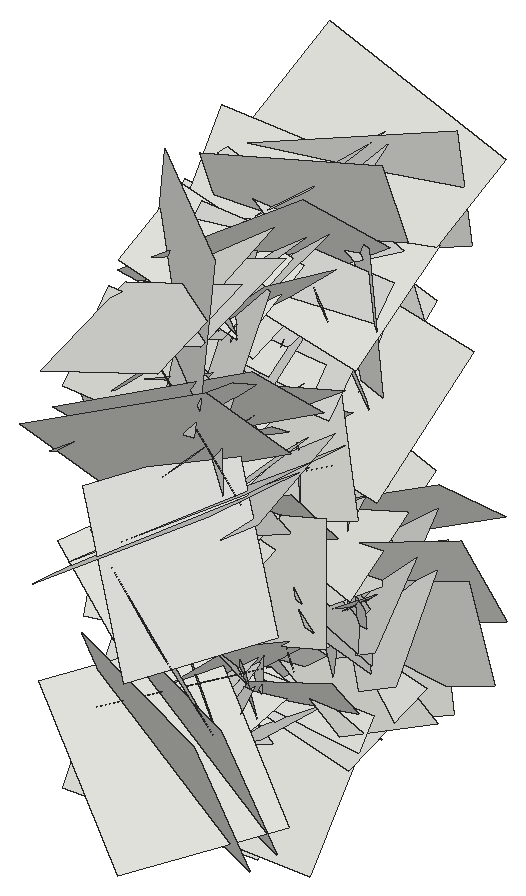
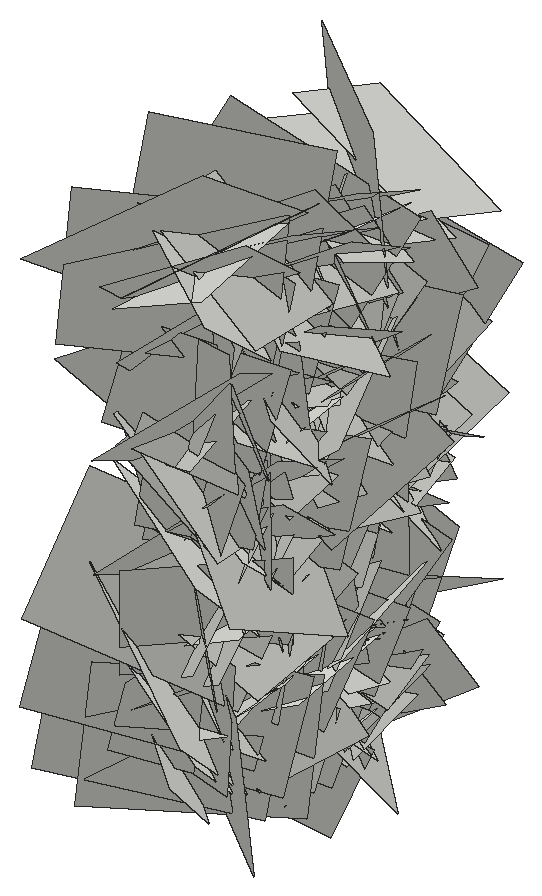
# SketchUp Ruby script. Lengths in inches.
U = 1.inch
M = Sketchup.active_model
def pt(a) = Geom::Point3d.new(a.map { |v| v * U })
def face(e, loops, mat)
  f = e.add_face(loops[0].map { |a| pt(a) })
  loops[1..].each { |l| e.add_face(l.map { |a| pt(a) }).erase! }
  f.material = f.back_material = mat if mat
  f
end
# faces: each face lists its corners as indices into pts; further lists are holes
def faces(e, pts, list, mat = nil) = list.each { |f| face(e, (f[0].is_a?(Array) ? f : [f]).map { |l| l.map { |i| pts[i] } }, mat) }
# xy, xz, yz: faces in a plane at the given z, y or x. An outline is a flat list of corners, or four numbers for a rectangle; further outlines are holes
def ring(l) = l.size == 4 ? [[l[0], l[1]], [l[2], l[1]], [l[2], l[3]], [l[0], l[3]]] : l.each_slice(2).to_a
def flat(e, list, mat, &to3) = list.each { |f| face(e, (f[0].is_a?(Array) ? f : [f]).map { |l| ring(l).map { |u, v| to3.(u, v) } }, mat) }
def xy(e, z, list, mat = nil) = flat(e, list, mat) { |x, y| [x, y, z] }
def xz(e, y, list, mat = nil) = flat(e, list, mat) { |x, z| [x, y, z] }
def yz(e, x, list, mat = nil) = flat(e, list, mat) { |y, z| [x, y, z] }
def lines(e, pts, list) = list.each { |a, b| e.add_line(pt(pts[a]), pt(pts[b])) }
# prism: a flat outline (further loops are holes) pulled along v
def prism(e, loops, v, mat = nil)
  f = face(e, loops, mat); d = Geom::Vector3d.new(v.map { |x| x * U })
  f.pushpull(f.normal.samedirection?(d) ? d.length : -d.length)
end
def box(e, o, s, mat = nil) = prism(e, [[o, [o[0] + s[0], o[1], o[2]], [o[0] + s[0], o[1] + s[1], o[2]], [o[0], o[1] + s[1], o[2]]]], [0, 0, s[2]], mat)
def at(x, y, z, deg = 0) = Geom::Transformation.translation(pt([x, y, z])) * Geom::Transformation.rotation(ORIGIN, Z_AXIS, deg.degrees)
def axes(o, x, y, z) = Geom::Transformation.new([*x, 0, *y, 0, *z, 0, *pt(o).to_a, 1])
def part(name) = M.definitions.add(name)
# library, detail: a bought-in or finely detailed component or shape, given as its bounding box
def library(name, o, s) = part(name).tap { |d| box(d.entities, o, s) }
def detail(e, o, s) = box(e.add_group.entities, o, s)
def put(e, d, t, mat = nil) = e.add_instance(d, t).tap { |i| i.material = mat if mat }
def group(e, t, mat = nil) = e.add_group.tap { |g| g.transformation = t; g.material = mat if mat }.entities
root = M.entities
c1 = part("Component\#6")
p = [[0.01,0,0],[0,3.24,4.54],[4.32,3.24,4.54],[4.33,0,0]]
faces(c1.entities,p,[[0,1,2,3]])
put(root,c1,axes([38.11,133.2,0.29],[0.16868,0.00753,1.30134],[0.16064,1.302,-0.02607],[-1.37005,0.15359,0.15716]))
put(root,c1,axes([34.14,134.57,7.51],[-0.06425,-0.0713,-0.65597],[0.02618,-0.65852,0.06929],[0.69893,0.01811,-0.0629]))
put(root,c1,axes([38.11,128.52,17.74],[-0.08604,0.43028,-0.81229],[-0.04293,-0.81633,-0.42838],[-0.97342,-0.00203,0.0907]))
put(root,c1,axes([34.14,132.11,13.83],[-0.12823,-0.67114,-0.46171],[-0.10246,-0.45164,0.68184],[0.85739,-0.15435,0.01243]))
put(root,c1,axes([38.11,133.79,15.82],[-0.11741,-0.82822,-0.37202],[-0.00882,-0.37384,0.83474],[-0.96237,0.10447,0.03774]))
put(root,c1,axes([34.14,131.53,3.64],[-0.03356,0.34972,-0.55611],[0.01458,-0.55628,-0.35061],[0.69619,0.02851,-0.01946]))
put(root,c1,axes([34.14,130.57,14.69],[-0.08088,0.56373,-0.36339],[0.06437,-0.35843,-0.56878],[0.70803,0.09698,0.0102]))
put(root,c1,axes([38.11,130.125,12.36],[0.14413,1.23778,0.56401],[0.30073,0.52855,-1.22835],[-1.41013,0.23923,-0.20431]))
put(root,c1,axes([38.11,129.28,18.375],[-0.15104,-0.37703,-0.77667],[0.00911,-0.78776,0.38083],[-0.9151,0.05438,0.13199]))
put(root,c1,axes([38.11,132.6,22.9],[-0.05818,0.99288,0.05669],[0.07779,0.06066,-0.99145],[-1.05129,-0.05046,-0.07649]))
put(root,c1,axes([34.14,133.3125,17.59],[0.01529,0.27468,0.5349],[0.08187,0.52978,-0.27413],[0.6321,-0.07526,0.02257]))
put(root,c1,axes([34.14,129.84,16.13],[0.05288,0.68465,0.04631],[-0.09068,0.05228,-0.68068],[0.72171,-0.04359,-0.08892]))
put(root,c1,axes([38.11,129.45,15.69],[0.00555,0.72683,0.86308],[0.19522,0.85097,-0.71774],[-1.18002,0.1442,-0.11468]))
put(root,c1,axes([34.14,129.41,10.95],[-0.18775,-0.48629,-0.69123],[0.00245,-0.70652,0.49646],[0.89586,-0.09998,-0.14623]))
put(root,c1,axes([34.14,132.63,6.14],[-0.10731,0.87556,-0.00554],[-0.12201,-0.01884,-0.87366],[0.92006,0.09962,-0.1165]))
put(root,c1,axes([38.11,133.96,12.5],[-0.03937,0.24323,0.81298],[-0.12274,0.80469,-0.24604],[-0.89109,-0.12158,-0.00203]))
put(root,c1,axes([38.11,127.6,6.32],[-0.09105,0.77875,-0.27248],[-0.08108,-0.28029,-0.77696],[-0.87078,-0.05533,0.10084]))
put(root,c1,axes([38.11,133.1,9.3125],[0.02086,0.87239,-0.16813],[-0.14049,-0.16341,-0.8634],[-0.93122,0.04419,0.12649]))
put(root,c1,axes([38.11,131.05,1.96],[0.03915,-1.05631,0.36623],[0.17317,0.36759,1.04378],[-1.17236,0.01903,0.16641]))
put(root,c1,axes([34.14,133.88,6.93],[-0.12434,-0.60409,0.41763],[0.12699,0.40152,0.61444],[0.76804,-0.16419,-0.03398]))
put(root,c1,axes([38.11,136.93,7.59],[0.11136,0.24127,-0.97313],[-0.07388,-0.97433,-0.24909],[-1.06018,0.09324,-0.08486]))
put(root,c1,axes([34.14,130.03,2.94],[-0.11679,-0.3481,0.76621],[-0.04914,0.77408,0.34502],[0.89071,-0.00294,0.1195]))
put(root,c1,axes([34.14,129.23,5.41],[-0.17398,-0.60139,0.60701],[0.02487,0.6147,0.61536],[0.9054,-0.13245,0.09973]))
put(root,c1,axes([38.11,132.5,3.06],[0.12033,-0.77552,-0.96336],[0.26418,-0.93322,0.78062],[-1.28404,-0.26468,0.07033]))
put(root,c1,axes([34.14,129.18,10.77],[0.08644,0.04023,-0.60323],[0.06997,-0.60565,-0.03147],[0.63702,0.06107,0.08531]))
put(root,c1,axes([38.11,132.55,10.48],[0.11298,-1.07137,-0.22101],[0.09706,-0.21254,1.07447],[-1.1555,-0.12261,0.06864]))
put(root,c1,axes([34.14,128.34,18.92],[0.04874,0.38349,0.62334],[-0.06251,0.62448,-0.37984],[0.77325,0.02631,-0.07]))
put(root,c1,axes([34.14,129.8,15.91],[0.05085,-0.71724,0.33006],[-0.13843,0.31891,0.71198],[0.82538,0.09767,0.09907]))
put(root,c1,axes([38.11,127.86,19.19],[0.25173,1.01088,0.57921],[0.04385,0.58343,-1.03521],[-1.23418,0.22691,0.08136]))
put(root,c1,axes([38.11,127.34,21.1],[0.03089,0.79811,0.32897],[-0.11706,0.3299,-0.79059],[-0.90753,-0.01539,0.11317]))
put(root,c1,axes([34.14,133.42,16.97],[-0.14677,0.94615,0.46149],[-0.22557,0.4307,-0.94687],[1.09283,0.21597,-0.13346]))
put(root,c1,axes([34.14,133.96,6.46],[-0.0893,0.11056,0.97068],[-0.19494,0.95507,-0.12474],[1.01706,0.19277,0.06132]))
put(root,c1,axes([38.11,136.53,11.26],[0.01536,-0.64622,-0.54667],[-0.11065,-0.54394,0.64022],[-0.89037,0.05645,-0.089]))
put(root,c1,axes([34.14,131.99,-0.9375],[0.0225,-0.54484,0.50649],[-0.02225,0.50605,0.54525],[0.78821,0.02984,0.00093]))
put(root,c1,axes([38.11,127.95,5.4],[-0.05879,0.74539,0.22064],[-0.10629,0.21249,-0.74307],[-0.81711,-0.08127,0.08079]))
put(root,c1,axes([34.14,125.86,8.82],[0.02658,0.53015,0.39509],[0.11889,0.38623,-0.52538],[0.69069,-0.08688,0.07523]))
put(root,c1,axes([34.14,131.86,3.01],[0.01467,-0.55248,-0.51034],[-0.00827,-0.51051,0.55244],[0.7972,0.00487,0.01512]))
put(root,c1,axes([34.14,136.82,15.87],[-0.16772,-0.74319,-0.48228],[0.03783,-0.49486,0.75087],[0.93836,-0.11289,-0.11647]))
put(root,c1,axes([38.11,125.93,11.7],[-0.16945,0.67455,-0.05214],[-0.09647,-0.07453,-0.68517],[-0.71064,-0.15073,0.10544]))
put(root,c1,axes([38.11,127.92,4.7],[-0.092,0.70183,0.2556],[-0.07294,0.24871,-0.70628],[-0.78837,-0.10491,0.03552]))
put(root,c1,axes([38.11,128.53,16.93],[0.30517,1.08519,-0.55956],[0.1011,-0.59314,-1.10124],[-1.29027,0.21019,-0.21864]))
put(root,c1,axes([34.14,137.37,4.77],[-0.01509,-0.67708,-0.46908],[-0.05072,-0.46768,0.67651],[0.87164,-0.03894,0.03124]))
put(root,c1,axes([38.11,133.14,16.06],[0.03738,-0.31853,0.81486],[-0.04959,0.81367,0.32009],[-0.92608,-0.05642,0.01575]))
put(root,c1,axes([38.11,133.58,20.74],[0.06025,0.71815,0.57437],[0.00066,0.57544,-0.71955],[-0.97476,0.04478,0.03501]))
put(root,c1,axes([38.11,131.35,15.19],[-0.02447,0.82058,-0.14823],[-0.01236,-0.14859,-0.82075],[-0.8838,-0.02064,0.01558]))
put(root,c1,axes([34.14,130.01,4.69],[0.05447,0.12092,0.77662],[-0.06993,0.77619,-0.11649],[0.83019,0.05744,-0.06077]))
put(root,c1,axes([38.11,135.14,15.06],[0.15738,0.18416,-1.10832],[0.16264,-1.1108,-0.16402],[-1.17977,-0.12857,-0.17046]))
put(root,c1,axes([38.11,133.07,14.74],[0.12706,0.28525,0.91315],[-0.02767,0.92092,-0.28425],[-1.01369,0.01061,0.12222]))
put(root,c1,axes([38.11,132.96,18.89],[0.10145,-0.91774,-0.17179],[-0.02227,-0.17476,0.92192],[-0.98945,-0.09016,-0.03837]))
put(root,c1,axes([34.14,135.65,2.32],[-0.1935,-1.06071,0.09437],[-0.13048,0.11613,1.0671],[1.12123,-0.16954,0.14047]))
put(root,c1,axes([34.14,136.42,13.64],[0.14309,-0.55174,0.41683],[-0.03038,0.41987,0.56505],[0.73236,0.12522,-0.058]))
put(root,c1,axes([38.11,137.27,19.36],[0.1763,0.15017,-0.9005],[-0.15684,-0.89878,-0.17721],[-0.95491,0.17535,-0.13715]))
put(root,c1,axes([38.11,130.2,1.79],[0.1042,-0.77086,0.73803],[0.17604,0.74317,0.75412],[-1.11745,0.04519,0.18762]))
put(root,c1,axes([38.11,136.01,11.51],[-0.06598,-0.27091,0.62957],[-0.16839,0.62065,0.25136],[-0.70672,-0.12259,-0.11867]))
put(root,c1,axes([34.14,133.51,8.98],[-0.15319,0.47062,-0.90401],[-0.09722,-0.91536,-0.46187],[1.07594,-0.0157,-0.17044]))
put(root,c1,axes([38.11,126.24,11.02],[-0.17433,0.41563,0.4957],[-0.04437,0.50356,-0.43611],[-0.68427,-0.13854,-0.09801]))
put(root,c1,axes([34.14,132.67,11.61],[-0.16439,-1.14375,-0.17253],[-0.24163,-0.14044,1.13591],[1.20204,-0.18465,0.20475]))
put(root,c1,axes([38.11,132.67,11.61],[0.16439,-1.14375,-0.17253],[0.24163,-0.14044,1.13591],[-1.20204,-0.18465,0.20475]))
put(root,c1,axes([34.14,126.24,11.02],[0.17433,0.41563,0.4957],[0.04437,0.50356,-0.43611],[0.68427,-0.13854,-0.09801]))
put(root,c1,axes([38.11,133.51,8.98],[0.15319,0.47062,-0.90401],[0.09722,-0.91536,-0.46187],[-1.07594,-0.0157,-0.17044]))
put(root,c1,axes([34.14,136.01,11.51],[0.06598,-0.27091,0.62957],[0.16839,0.62065,0.25136],[0.70672,-0.12259,-0.11867]))
put(root,c1,axes([34.14,130.2,1.79],[-0.1042,-0.77086,0.73803],[-0.17604,0.74317,0.75412],[1.11745,0.04519,0.18762]))
put(root,c1,axes([34.14,137.27,19.36],[-0.1763,0.15017,-0.9005],[0.15684,-0.89878,-0.17721],[0.95491,0.17535,-0.13715]))
put(root,c1,axes([38.11,136.42,13.64],[-0.14309,-0.55174,0.41683],[0.03038,0.41987,0.56505],[-0.73236,0.12522,-0.058]))
put(root,c1,axes([38.11,135.65,2.32],[0.1935,-1.06071,0.09437],[0.13048,0.11613,1.0671],[-1.12123,-0.16954,0.14047]))
put(root,c1,axes([34.14,132.96,18.89],[-0.10145,-0.91774,-0.17179],[0.02227,-0.17476,0.92192],[0.98945,-0.09016,-0.03837]))
put(root,c1,axes([34.14,133.07,14.74],[-0.12706,0.28525,0.91315],[0.02767,0.92092,-0.28425],[1.01369,0.01061,0.12222]))
put(root,c1,axes([34.14,135.14,15.06],[-0.15738,0.18416,-1.10832],[-0.16264,-1.1108,-0.16402],[1.17977,-0.12857,-0.17046]))
put(root,c1,axes([38.11,130.01,4.69],[-0.05447,0.12092,0.77662],[0.06993,0.77619,-0.11649],[-0.83019,0.05744,-0.06077]))
put(root,c1,axes([34.14,131.35,15.19],[0.02447,0.82058,-0.14823],[0.01236,-0.14859,-0.82075],[0.8838,-0.02064,0.01558]))
put(root,c1,axes([34.14,133.58,20.74],[-0.06025,0.71815,0.57437],[-0.00066,0.57544,-0.71955],[0.97476,0.04478,0.03501]))
put(root,c1,axes([34.14,133.14,16.06],[-0.03738,-0.31853,0.81486],[0.04959,0.81367,0.32009],[0.92608,-0.05642,0.01575]))
put(root,c1,axes([38.11,137.37,4.77],[0.01509,-0.67708,-0.46908],[0.05072,-0.46768,0.67651],[-0.87164,-0.03894,0.03124]))
put(root,c1,axes([34.14,128.53,16.93],[-0.30517,1.08519,-0.55956],[-0.1011,-0.59314,-1.10124],[1.29027,0.21019,-0.21864]))
put(root,c1,axes([34.14,127.92,4.7],[0.092,0.70183,0.2556],[0.07294,0.24871,-0.70628],[0.78837,-0.10491,0.03552]))
put(root,c1,axes([34.14,125.93,11.7],[0.16945,0.67455,-0.05214],[0.09647,-0.07453,-0.68517],[0.71064,-0.15073,0.10544]))
put(root,c1,axes([38.11,136.82,15.87],[0.16772,-0.74319,-0.48228],[-0.03783,-0.49486,0.75087],[-0.93836,-0.11289,-0.11647]))
put(root,c1,axes([38.11,131.86,3.01],[-0.01467,-0.55248,-0.51034],[0.00827,-0.51051,0.55244],[-0.7972,0.00487,0.01512]))
put(root,c1,axes([38.11,125.86,8.82],[-0.02658,0.53015,0.39509],[-0.11889,0.38623,-0.52538],[-0.69069,-0.08688,0.07523]))
put(root,c1,axes([34.14,127.95,5.4],[0.05879,0.74539,0.22064],[0.10629,0.21249,-0.74307],[0.81711,-0.08127,0.08079]))
put(root,c1,axes([38.11,131.99,-0.9375],[-0.0225,-0.54484,0.50649],[0.02225,0.50605,0.54525],[-0.78821,0.02984,0.00093]))
put(root,c1,axes([34.14,136.53,11.26],[-0.01536,-0.64622,-0.54667],[0.11065,-0.54394,0.64022],[0.89037,0.05645,-0.089]))
put(root,c1,axes([38.11,133.96,6.46],[0.0893,0.11056,0.97068],[0.19494,0.95507,-0.12474],[-1.01706,0.19277,0.06132]))
put(root,c1,axes([34.14,127.34,21.1],[-0.03089,0.79811,0.32897],[0.11706,0.3299,-0.79059],[0.90753,-0.01539,0.11317]))
put(root,c1,axes([34.14,127.86,19.19],[-0.25173,1.01088,0.57921],[-0.04385,0.58343,-1.03521],[1.23418,0.22691,0.08136]))
put(root,c1,axes([38.11,129.8,15.91],[-0.05085,-0.71724,0.33006],[0.13843,0.31891,0.71198],[-0.82538,0.09767,0.09907]))
put(root,c1,axes([38.11,128.34,18.92],[-0.04874,0.38349,0.62334],[0.06251,0.62448,-0.37984],[-0.77325,0.02631,-0.07]))
put(root,c1,axes([34.14,132.55,10.48],[-0.11298,-1.07137,-0.22101],[-0.09706,-0.21254,1.07447],[1.1555,-0.12261,0.06864]))
put(root,c1,axes([38.11,129.18,10.77],[-0.08644,0.04023,-0.60323],[-0.06997,-0.60565,-0.03147],[-0.63702,0.06107,0.08531]))
put(root,c1,axes([34.14,132.5,3.06],[-0.12033,-0.77552,-0.96336],[-0.26418,-0.93322,0.78062],[1.28404,-0.26468,0.07033]))
put(root,c1,axes([38.11,129.23,5.41],[0.17398,-0.60139,0.60701],[-0.02487,0.6147,0.61536],[-0.9054,-0.13245,0.09973]))
put(root,c1,axes([38.11,130.03,2.94],[0.11679,-0.3481,0.76621],[0.04914,0.77408,0.34502],[-0.89071,-0.00294,0.1195]))
put(root,c1,axes([34.14,136.93,7.59],[-0.11136,0.24127,-0.97313],[0.07388,-0.97433,-0.24909],[1.06018,0.09324,-0.08486]))
put(root,c1,axes([38.11,133.88,6.93],[0.12434,-0.60409,0.41763],[-0.12699,0.40152,0.61444],[-0.76804,-0.16419,-0.03398]))
put(root,c1,axes([34.14,131.05,1.96],[-0.03915,-1.05631,0.36623],[-0.17317,0.36759,1.04378],[1.17236,0.01903,0.16641]))
put(root,c1,axes([34.14,133.1,9.3125],[-0.02086,0.87239,-0.16813],[0.14049,-0.16341,-0.8634],[0.93122,0.04419,0.12649]))
put(root,c1,axes([34.14,127.6,6.32],[0.09105,0.77875,-0.27248],[0.08108,-0.28029,-0.77696],[0.87078,-0.05533,0.10084]))
put(root,c1,axes([34.14,133.96,12.5],[0.03937,0.24323,0.81298],[0.12274,0.80469,-0.24604],[0.89109,-0.12158,-0.00203]))
put(root,c1,axes([38.11,132.63,6.14],[0.10731,0.87556,-0.00554],[0.12201,-0.01884,-0.87366],[-0.92006,0.09962,-0.1165]))
put(root,c1,axes([38.11,129.41,10.95],[0.18775,-0.48629,-0.69123],[-0.00245,-0.70652,0.49646],[-0.89586,-0.09998,-0.14623]))
put(root,c1,axes([34.14,129.45,15.69],[-0.00555,0.72683,0.86308],[-0.19522,0.85097,-0.71774],[1.18002,0.1442,-0.11468]))
put(root,c1,axes([38.11,129.84,16.13],[-0.05288,0.68465,0.04631],[0.09068,0.05228,-0.68068],[-0.72171,-0.04359,-0.08892]))
put(root,c1,axes([38.11,133.3125,17.59],[-0.01529,0.27468,0.5349],[-0.08187,0.52978,-0.27413],[-0.6321,-0.07526,0.02257]))
put(root,c1,axes([34.14,132.6,22.9],[0.05818,0.99288,0.05669],[-0.07779,0.06066,-0.99145],[1.05129,-0.05046,-0.07649]))
put(root,c1,axes([34.14,129.28,18.375],[0.15104,-0.37703,-0.77667],[-0.00911,-0.78776,0.38083],[0.9151,0.05438,0.13199]))
put(root,c1,axes([34.14,130.125,12.36],[-0.14413,1.23778,0.56401],[-0.30073,0.52855,-1.22835],[1.41013,0.23923,-0.20431]))
put(root,c1,axes([38.11,130.57,14.69],[0.08088,0.56373,-0.36339],[-0.06437,-0.35843,-0.56878],[-0.70803,0.09698,0.0102]))
put(root,c1,axes([38.11,131.53,3.64],[0.03356,0.34972,-0.55611],[-0.01458,-0.55628,-0.35061],[-0.69619,0.02851,-0.01946]))
put(root,c1,axes([34.14,133.79,15.82],[0.11741,-0.82822,-0.37202],[0.00882,-0.37384,0.83474],[0.96237,0.10447,0.03774]))
put(root,c1,axes([38.11,132.11,13.83],[0.12823,-0.67114,-0.46171],[0.10246,-0.45164,0.68184],[-0.85739,-0.15435,0.01243]))
put(root,c1,axes([34.14,128.52,17.74],[0.08604,0.43028,-0.81229],[0.04293,-0.81633,-0.42838],[0.97342,-0.00203,0.0907]))
put(root,c1,axes([38.11,134.57,7.51],[0.06425,-0.0713,-0.65597],[-0.02618,-0.65852,0.06929],[-0.69893,0.01811,-0.0629]))
put(root,c1,axes([34.14,133.2,0.29],[-0.16868,0.00753,1.30134],[-0.16064,1.302,-0.02607],[1.37005,0.15359,0.15716]))
put(root,c1,axes([38.11,127.28,0.51],[0.04452,-0.40985,0.5808],[0.07759,0.58122,0.40485],[-0.7495,0.03582,0.07641]))
put(root,c1,axes([34.14,129.68,16.21],[0.16446,-0.17941,-0.82447],[0.07006,-0.83314,0.19373],[0.89165,0.09856,0.13685]))
put(root,c1,axes([38.11,134.26,15.51],[0.13639,0.72841,-0.25059],[0.07067,-0.26364,-0.7321],[-0.81346,0.09922,-0.10562]))
put(root,c1,axes([34.14,128.87,2.92],[0.01411,0.95221,-0.19006],[0.11482,-0.19035,-0.94606],[1.02282,0.00823,0.10882]))
put(root,c1,axes([34.14,138.97,11.375],[-0.02639,-0.72989,-0.72722],[0.07911,-0.7268,0.72691],[1.08928,0.0351,-0.07041]))
put(root,c1,axes([34.14,131.74,20.5625],[-0.11289,-0.41624,-1.03402],[0.06809,-1.03929,0.41174],[1.17957,0.02016,-0.12272]))
put(root,c1,axes([38.11,131.9,7.66],[0.03371,0.19161,0.61883],[0.06203,0.6162,-0.1938],[-0.68388,0.06533,0.01292]))
put(root,c1,axes([34.14,134.95,12.42],[0.03363,0.92541,-1.00089],[-0.39451,-0.95725,-0.89685],[1.39004,-0.29406,-0.23032]))
put(root,c1,axes([38.11,131.8,8.64],[0.08497,0.05507,0.67491],[0.04101,0.67814,-0.05993],[-0.71661,0.04534,0.0766]))
put(root,c1,axes([34.14,137.87,11.82],[0.23548,-0.98581,-0.19043],[-0.17104,-0.22756,0.98976],[1.05044,0.18394,0.20385]))
put(root,c1,axes([34.14,129.625,19.87],[-0.14331,0.9196,0.97349],[-0.15794,0.96203,-0.92947],[1.41069,0.20113,-0.00516]))
put(root,c1,axes([34.14,130.99,8.6],[0.04494,-0.64922,0.68663],[0.20873,0.6783,0.62918],[0.97967,-0.11474,-0.16555]))
put(root,c1,axes([34.14,133.91,11.1875],[-0.02059,0.92356,-0.8814],[-0.20413,-0.87353,-0.91107],[1.33776,-0.11908,-0.15259]))
put(root,c1,axes([34.14,128.56,10.3125],[-0.23413,0.04823,1.24691],[0.1221,1.26168,-0.02839],[1.31707,-0.10839,0.22429]))
put(root,c1,axes([34.14,131.94,16.85],[-0.08825,-0.96476,0.81898],[-0.08011,0.82307,0.9619],[1.33903,-0.01434,0.11152]))
put(root,c1,axes([34.14,131.18,15.16],[0.15294,-1.16278,0.39158],[-0.28955,0.35393,1.15166],[1.26792,0.22109,0.21577]))
put(root,c1,axes([38.11,134.77,2.57],[0.05447,0.40704,0.46107],[0.08155,0.45478,-0.41007],[-0.64681,0.09162,-0.01288]))
put(root,c1,axes([34.14,134.14,22.88],[0.03825,0.99518,-0.25742],[0.13842,-0.25993,-0.98657],[1.08078,-0.00193,0.13547]))
put(root,c1,axes([33.43,124.93,11.12],[0.54058,0.75668,0.32998],[0.30141,0.20311,-0.90522],[0.82148,-0.57246,0.11499]))
put(root,c1,axes([34.14,127.92,6.47],[-0.03611,0.05394,1.13531],[0.09971,1.13206,-0.05096],[1.20066,-0.09239,0.03838]))
put(root,c1,axes([38.11,138.1,17.99],[0.00934,-0.49027,-0.41508],[0.1892,-0.3969,0.47259],[-0.65411,-0.1218,0.13076]))
put(root,c1,axes([34.14,127.69,20.12],[-0.02742,-1.01137,-0.35231],[0.21232,-0.35076,0.99222],[1.1152,0.04191,-0.19757]))
put(root,c1,axes([34.14,130,20.12],[-0.02742,-1.01137,-0.35231],[0.21232,-0.35076,0.99222],[1.1152,0.04191,-0.19757]))
put(root,c1,axes([38.11,129.35,18.22],[0.07955,-0.40219,0.442],[0.06566,0.44831,0.39741],[-0.63004,-0.00406,0.09723]))
put(root,c1,axes([34.14,129.81,24.32],[-0.08615,-0.07511,-1.33483],[-0.12267,-1.33188,0.08199],[1.41184,-0.12031,-0.07433]))
put(root,c1,axes([34.14,131.16,1.32],[0.11103,-1.00768,0.14491],[0.13016,0.15712,1.00381],[1.07125,0.08535,-0.13699]))
put(root,c1,axes([34.14,136.29,19.65],[0.239,0.33681,-1.04778],[-0.13934,-1.05364,-0.36698],[1.15826,-0.19625,0.17205]))
put(root,c1,axes([34.14,129.42,5.47],[-0.26825,1.30607,0.06413],[0.25565,0.11082,-1.30519],[1.36232,0.23638,0.25756]))
put(root,c1,axes([34.14,126.61,12.8],[-0.1414,-0.87971,0.87765],[0.19082,0.8597,0.88908],[1.30331,-0.22132,-0.03495]))
put(root,c1,axes([34.14,133.96,9.66],[0.06967,-1.04066,0.34132],[0.1454,0.34706,1.03175],[1.15177,0.01914,-0.15089]))
put(root,c1,axes([34.14,134.94,17.85],[0.08672,-0.29938,1.1859],[-0.04442,1.18717,0.30259],[1.29573,0.06074,-0.069]))
put(root,c1,axes([34.14,129.48,20.64],[-0.14207,1.22324,0.51937],[0.11373,0.53026,-1.2212],[1.40407,0.08082,0.15147]))
put(root,c1,axes([34.14,129.66,12.47],[-0.1081,-1.2535,0.58167],[-0.00417,0.58351,1.25678],[1.46479,-0.09085,0.0465]))
put(root,c1,axes([34.14,125.82,11.42],[0.20547,0.4933,-0.99975],[0.03886,-1.01702,-0.49472],[1.18108,-0.05236,0.1902]))
put(root,c1,axes([34.14,131.95,0.87],[0.07095,-0.70744,0.83659],[0.30432,0.82019,0.6706],[1.12076,-0.17792,-0.23504]))
put(root,c1,axes([34.14,139.8125,5.82],[0.12038,-0.94885,-0.86303],[-0.08352,-0.86993,0.94607],[1.35702,0.03063,0.13479]))
put(root,c1,axes([34.14,133.04,19.75],[0.14526,-0.49923,0.95494],[0.24012,0.95446,0.46647],[1.11669,-0.1403,-0.22453]))
put(root,c1,axes([34.14,128.24,17.68],[0.22785,0.52614,1.07761],[-0.06777,1.09826,-0.52347],[1.26934,-0.03581,-0.22138]))
put(root,c1,axes([34.14,133.15,22.79],[0.15509,1.06813,0.73269],[-0.10614,0.74447,-1.06531],[1.36888,-0.06329,-0.16562]))
put(root,c1,axes([34.14,132.12,7.08],[-0.00585,1.22451,-0.43101],[0.11167,-0.42917,-1.22063],[1.3715,0.04016,0.09755]))
put(root,c1,axes([34.14,125.99,1.35],[0.00241,0.79041,1.08039],[0.06651,1.07914,-0.78963],[1.41741,-0.05198,0.03522]))
put(root,c1,axes([34.14,127.67,13.74],[0.06329,-0.97705,0.81505],[0.12838,0.8166,0.97005],[1.34259,-0.03203,-0.13118]))
put(root,c1,axes([34.14,137,19.49],[0.23927,-0.1296,-1.18474],[0.04055,-1.20439,0.13904],[1.26266,0.06324,0.22004]))
put(root,c1,axes([34.14,135.39,1.18],[0.01455,-0.40823,1.27358],[0.1801,1.26386,0.40328],[1.40617,-0.15765,-0.06483]))
put(root,c1,axes([34.14,128.0625,10.23],[0.10909,-1.3698,0.20566],[-0.00727,0.20572,1.37363],[1.46824,0.1028,-0.00848]))
put(root,c1,axes([34.14,129.98,10.23],[0.10909,-1.3698,0.20566],[-0.00727,0.20572,1.37363],[1.46824,0.1028,-0.00848]))
put(root,c1,axes([34.14,138.98,4.78],[0.22268,-0.9196,-0.8307],[0.07298,-0.83259,0.9391],[1.31157,0.20246,0.08879]))
put(root,c1,axes([32.97,124.5,5.79],[0.83668,1.07369,0.2523],[0.21003,0.16716,-1.33127],[1.15009,-0.81162,0.05958]))
put(root,c1,axes([34.14,130.78,10.54],[0.24762,-1.26357,-0.1726],[-0.00687,-0.17664,1.28442],[1.3518,0.23056,0.03815]))
put(root,c1,axes([34.14,136.82,5.83],[0.1656,-1.02965,0.80161],[0.14776,0.81588,1.02082],[1.37528,0.03632,-0.2062]))
put(root,c1,axes([34.14,130.15,15.41],[0.24379,0.89731,1.03665],[0.02149,1.04879,-0.91232],[1.45316,-0.16605,-0.16042]))
put(root,c1,axes([34.14,135.96,3.29],[0.1622,-0.76384,1.11136],[0.23079,1.11781,0.7383],[1.4107,-0.09505,-0.24857]))
put(root,c1,axes([34.14,125.3125,7.6875],[0.15543,0.49215,-1.26812],[0.29157,-1.25984,-0.45713],[1.41209,0.20597,0.23397]))
put(root,c1,axes([34.14,126.76,7.6875],[0.15543,0.49215,-1.26812],[0.29157,-1.25984,-0.45713],[1.41209,0.20597,0.23397]))
put(root,c1,axes([34.04,125.5,13.2],[1.07209,0.56535,0.5401],[0.40295,0.41611,-1.14744],[0.72423,-1.06841,-0.1611]))
